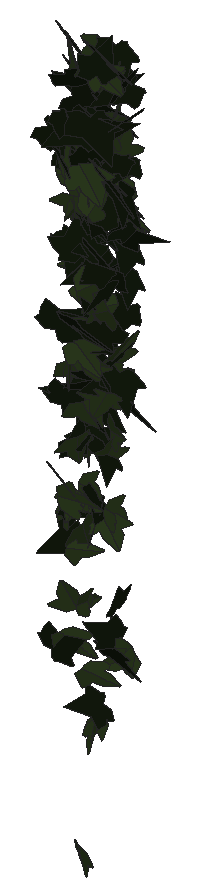
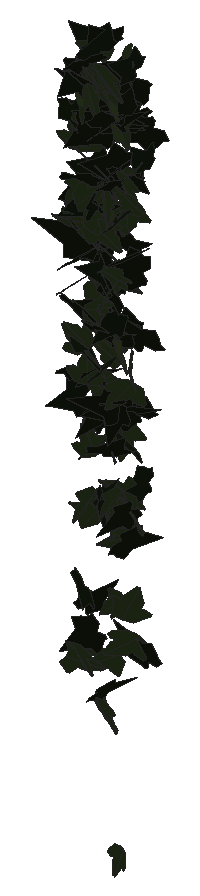
# SketchUp Ruby script. Lengths in inches.
U = 1.inch
M = Sketchup.active_model
def pt(a) = Geom::Point3d.new(a.map { |v| v * U })
def face(e, loops, mat)
  f = e.add_face(loops[0].map { |a| pt(a) })
  loops[1..].each { |l| e.add_face(l.map { |a| pt(a) }).erase! }
  f.material = f.back_material = mat if mat
  f
end
# faces: each face lists its corners as indices into pts; further lists are holes
def faces(e, pts, list, mat = nil) = list.each { |f| face(e, (f[0].is_a?(Array) ? f : [f]).map { |l| l.map { |i| pts[i] } }, mat) }
# xy, xz, yz: faces in a plane at the given z, y or x. An outline is a flat list of corners, or four numbers for a rectangle; further outlines are holes
def ring(l) = l.size == 4 ? [[l[0], l[1]], [l[2], l[1]], [l[2], l[3]], [l[0], l[3]]] : l.each_slice(2).to_a
def flat(e, list, mat, &to3) = list.each { |f| face(e, (f[0].is_a?(Array) ? f : [f]).map { |l| ring(l).map { |u, v| to3.(u, v) } }, mat) }
def xy(e, z, list, mat = nil) = flat(e, list, mat) { |x, y| [x, y, z] }
def xz(e, y, list, mat = nil) = flat(e, list, mat) { |x, z| [x, y, z] }
def yz(e, x, list, mat = nil) = flat(e, list, mat) { |y, z| [x, y, z] }
def lines(e, pts, list) = list.each { |a, b| e.add_line(pt(pts[a]), pt(pts[b])) }
# prism: a flat outline (further loops are holes) pulled along v
def prism(e, loops, v, mat = nil)
  f = face(e, loops, mat); d = Geom::Vector3d.new(v.map { |x| x * U })
  f.pushpull(f.normal.samedirection?(d) ? d.length : -d.length)
end
def box(e, o, s, mat = nil) = prism(e, [[o, [o[0] + s[0], o[1], o[2]], [o[0] + s[0], o[1] + s[1], o[2]], [o[0], o[1] + s[1], o[2]]]], [0, 0, s[2]], mat)
def at(x, y, z, deg = 0) = Geom::Transformation.translation(pt([x, y, z])) * Geom::Transformation.rotation(ORIGIN, Z_AXIS, deg.degrees)
def axes(o, x, y, z) = Geom::Transformation.new([*x, 0, *y, 0, *z, 0, *pt(o).to_a, 1])
def part(name) = M.definitions.add(name)
# library, detail: a bought-in or finely detailed component or shape, given as its bounding box
def library(name, o, s) = part(name).tap { |d| box(d.entities, o, s) }
def detail(e, o, s) = box(e.add_group.entities, o, s)
def put(e, d, t, mat = nil) = e.add_instance(d, t).tap { |i| i.material = mat if mat }
def group(e, t, mat = nil) = e.add_group.tap { |g| g.transformation = t; g.material = mat if mat }.entities
root = M.entities
M.materials.add("1026 AP 7946 SUNNY SIDE UP").color = [254, 231, 186]
M.materials.add("efeu1").color = [18, 25, 13]
M.materials.add("efeu2").color = [43, 57, 29]
c1 = part("ivyleaf_9")
p = [[1.54,2.16,1.25],[1.36,2.04,1.19],[-0.21,0.99,0.68],[-0.71,1.11,0.82],[-0.85,0.86,0.67],[-0.8,0.17,0.21],
  [-0.9,-0.01,0.1],[-0.67,-0.16,-0.02],[-0.08,-0.08,-0.05],[-0.03,-0.6,-0.4],[0.65,-0.88,-0.66],[0.83,-0.6,-0.49],
  [1.29,-0.42,-0.43],[1.8125,-0.07,-0.26],[1.21,0.44,0.15]]
faces(c1.entities,p,[[0,1,2,3,4,5,6,7,8,9,10,11,12,13,14]],"efeu1")
c2 = part("ivyleaf_10")
p = [[0,0.5,-0.03],[-0.0625,2.02,-0.43],[-0.19,2.01,-0.46],[-0.54,1.05,-0.29],[-0.52,0.625,-0.18],[-0.83,0.76,-0.28],
  [-1.16,0.64,-0.33],[-1.15,0.33,-0.24],[-0.77,-0.39,0.02],[-0.3,-0.51,0.16],[0.04,-0.48,0.23],[-0.02,2.01,-0.4375],
  [-0.06,2.01,-0.43],[0.04,-0.49,0.23],[0.67,-0.49,0.14],[1.38,0.36,-0.2],[1.375,0.51,-0.24],[0.81,0.65,-0.19],
  [0.62,0.59,-0.15],[0.6,1.09,-0.28],[0.5,1.23,-0.31]]
faces(c2.entities,p,[[0,1,2,3,4,5,6,7,8,9,10],[11,12,0,13,14,15,16,17,18,19,20]],"efeu2")
put(root,c1,axes([113.27,211.88,254.59],[-0.05004,0.07467,0.25813],[0.2583,-0.19012,0.07888],[0.31902,0.16565,-0.02338]),"1026 AP 7946 SUNNY SIDE UP")
put(root,c2,axes([113.63,212.07,255.59],[-0.29468,-0.15309,-0.11384],[-0.15695,-0.0504,0.24797],[-0.25106,0.21119,-0.0214]),"1026 AP 7946 SUNNY SIDE UP")
put(root,c2,axes([113.6,212.22,265.22],[0.30589,-0.1507,-0.09853],[-0.12709,0.05033,-0.25304],[0.24942,0.21047,-0.0081]),"1026 AP 7946 SUNNY SIDE UP")
put(root,c1,axes([113.29,211.87,258.46],[0.30159,-0.16187,0.03135],[0.01844,-0.03457,-0.25804],[0.25859,0.19124,-0.01816]),"1026 AP 7946 SUNNY SIDE UP")
put(root,c1,axes([113.3,211.93,265.42],[0.08383,-0.17841,0.21618],[0.07856,-0.20497,-0.19289],[0.42714,0.07271,-0.00695]),"1026 AP 7946 SUNNY SIDE UP")
put(root,c1,axes([113.27,212.27,267.75],[0.20315,-0.19062,0.11843],[0.08131,-0.10486,-0.23738],[0.34134,0.13843,-0.01394]),"1026 AP 7946 SUNNY SIDE UP")
put(root,c2,axes([113.24,212.27,264.72],[0.22167,-0.09358,-0.21902],[0.3188,-0.07055,0.1705],[-0.17669,-0.24469,0.03285]),"1026 AP 7946 SUNNY SIDE UP")
put(root,c2,axes([113.625,211.9,265.02],[-0.03111,0.21778,-0.19952],[-0.04804,0.19274,0.22618],[0.45703,0.03508,0.0102]),"1026 AP 7946 SUNNY SIDE UP")
put(root,c2,axes([113.45,212.23,260.65],[-0.26135,-0.14427,-0.15787],[0.19582,0.08871,-0.22588],[0.26564,-0.20734,0.01119]),"1026 AP 7946 SUNNY SIDE UP")
put(root,c1,axes([113.78,212.56,266.45],[-0.05787,0.05868,0.25753],[-0.38787,-0.07709,-0.01925],[0.11031,-0.24029,0.06743]),"1026 AP 7946 SUNNY SIDE UP")
put(root,c2,axes([113.59,212.34,266.46],[0.02658,-0.25701,0.0449],[-0.0011,-0.04518,-0.26558],[0.41028,0.01653,-0.00362]),"1026 AP 7946 SUNNY SIDE UP")
put(root,c1,axes([113.34,211.91,261.54],[-0.15864,0.08613,0.25559],[0.34664,-0.11572,0.13333],[0.2231,0.24104,-0.02541]),"1026 AP 7946 SUNNY SIDE UP")
put(root,c1,axes([113.82,212.31,260.06],[-0.21043,-0.00737,0.21983],[-0.31368,-0.08559,-0.1324],[0.11986,-0.23693,0.03943]),"1026 AP 7946 SUNNY SIDE UP")
put(root,c1,axes([113.5,212.7,265.54],[-0.06622,-0.20645,0.13706],[-0.03746,-0.1321,-0.21782],[0.38537,-0.04832,0.00238]),"1026 AP 7946 SUNNY SIDE UP")
put(root,c2,axes([113.37,212.01,257.55],[0.11479,-0.15018,-0.19142],[0.19594,-0.14081,0.16763],[-0.3193,-0.1404,0.03405]),"1026 AP 7946 SUNNY SIDE UP")
put(root,c2,axes([113.63,212.33,261.53],[0.16132,-0.2266,-0.02126],[-0.03401,0.0114,-0.25572],[0.35598,0.10378,-0.0148]),"1026 AP 7946 SUNNY SIDE UP")
put(root,c1,axes([113.27,212.07,263.2],[0.30243,-0.1217,0.14574],[0.168,-0.09595,-0.2341],[0.24157,0.21908,-0.01965]),"1026 AP 7946 SUNNY SIDE UP")
put(root,c1,axes([113.36,212.45,266.84],[0.09024,-0.15114,0.22857],[0.14243,-0.2036,-0.16757],[0.39855,0.10699,0.00813]),"1026 AP 7946 SUNNY SIDE UP")
put(root,c1,axes([113.45,212.53,264.46],[0.06337,-0.24092,0.07907],[0.02803,-0.07621,-0.25204],[0.39726,0.04381,0.00517]),"1026 AP 7946 SUNNY SIDE UP")
put(root,c1,axes([113.42,211.57,266.09],[0.06896,0.01598,-0.27906],[0.08466,0.26852,0.02686],[0.41833,-0.05697,0.04056]),"1026 AP 7946 SUNNY SIDE UP")
put(root,c1,axes([113.64,212.37,260.22],[0.31328,-0.00666,-0.15655],[-0.23905,-0.01452,-0.20482],[-0.00554,0.25013,-0.01459]),"1026 AP 7946 SUNNY SIDE UP")
put(root,c1,axes([113.7,212.05,257.125],[0.00686,-0.10836,-0.27003],[0.09102,-0.25566,0.10864],[-0.43568,-0.05512,0.01845]),"1026 AP 7946 SUNNY SIDE UP")
put(root,c2,axes([113.84,211.79,267.53],[-0.08352,0.08772,-0.29124],[-0.17598,0.2605,0.10627],[0.43169,0.12316,-0.01303]),"1026 AP 7946 SUNNY SIDE UP")
put(root,c2,axes([113.7,212,264.4],[-0.37137,-0.10293,-0.00003],[0.01359,-0.02122,-0.26449],[0.16127,-0.23523,0.02222]),"1026 AP 7946 SUNNY SIDE UP")
put(root,c2,axes([113.9375,212.17,262.93],[-0.10002,0.0419,0.23465],[-0.34842,-0.07891,-0.0493],[0.10464,-0.22269,0.06011]),"1026 AP 7946 SUNNY SIDE UP")
put(root,c1,axes([113.6,212,257.8],[0.07037,-0.02062,-0.25548],[-0.11456,0.23972,-0.03269],[0.37396,0.07732,0.03806]),"1026 AP 7946 SUNNY SIDE UP")
put(root,c1,axes([113.62,212.17,263.4],[-0.13101,-0.22908,0.09166],[-0.0102,-0.09322,-0.25043],[0.38703,-0.08,0.02442]),"1026 AP 7946 SUNNY SIDE UP")
put(root,c2,axes([113.61,212.18,264.29],[-0.01572,-0.05606,0.26335],[0.14029,-0.24155,-0.05233],[0.38737,0.08521,0.02964]),"1026 AP 7946 SUNNY SIDE UP")
put(root,c1,axes([113.56,212.19,265.27],[-0.21319,-0.11264,-0.17533],[0.22079,0.09573,-0.18064],[0.23172,-0.19485,0.01081]),"1026 AP 7946 SUNNY SIDE UP")
put(root,c2,axes([113.65,212.4375,266.98],[0.13269,-0.19606,0.17999],[0.08969,-0.16664,-0.2206],[0.40426,0.10132,-0.01014]),"1026 AP 7946 SUNNY SIDE UP")
put(root,c2,axes([113.52,212.03,260.88],[0.13338,-0.1309,0.24849],[0.25586,-0.18027,-0.1603],[0.34875,0.18231,0.02257]),"1026 AP 7946 SUNNY SIDE UP")
put(root,c1,axes([113.58,212.3,265.2],[-0.03379,-0.28354,-0.06617],[0.01587,0.06202,-0.29252],[0.4563,-0.02315,0.00527]),"1026 AP 7946 SUNNY SIDE UP")
put(root,c1,axes([113.48,211.91,259.96],[-0.08664,0.04162,0.2526],[0.34837,-0.10536,0.06917],[0.17688,0.22791,-0.01249]),"1026 AP 7946 SUNNY SIDE UP")
put(root,c2,axes([113.75,212.52,264.82],[0.06468,-0.23733,-0.09699],[0.00366,0.09435,-0.24696],[0.40068,0.03745,0.01791]),"1026 AP 7946 SUNNY SIDE UP")
put(root,c1,axes([113.5,212.12,260.1],[0.22925,0.09403,0.21067],[0.27717,0.10278,-0.17802],[-0.21884,0.22867,-0.00478]),"1026 AP 7946 SUNNY SIDE UP")
put(root,c2,axes([113.92,212.59,264.17],[-0.25604,-0.09566,0.17523],[-0.19915,-0.11765,-0.19315],[0.23442,-0.20443,0.02731]),"1026 AP 7946 SUNNY SIDE UP")
put(root,c1,axes([113.84,211.79,259.18],[-0.27709,0.15901,-0.09797],[-0.09756,0.07434,0.24461],[0.27529,0.1864,-0.01192]),"1026 AP 7946 SUNNY SIDE UP")
put(root,c1,axes([113.64,211.69,266.43],[0.10789,-0.08843,-0.24258],[-0.09764,0.23004,-0.10652],[0.3825,0.08367,0.04123]),"1026 AP 7946 SUNNY SIDE UP")
put(root,c2,axes([113.57,211.9375,254.93],[-0.27349,-0.07845,-0.18939],[0.2844,0.04058,-0.19436],[0.13226,-0.24948,0.0263]),"1026 AP 7946 SUNNY SIDE UP")
put(root,c2,axes([113.75,212.11,250.25],[-0.27635,0.16463,-0.00203],[-0.01617,-0.01522,-0.24747],[-0.2584,-0.17511,0.01766]),"1026 AP 7946 SUNNY SIDE UP")
put(root,c2,axes([113.92,212.48,267.57],[0.31323,-0.13901,-0.15376],[-0.2093,0.06801,-0.2492],[0.24179,0.23895,-0.01653]),"1026 AP 7946 SUNNY SIDE UP")
put(root,c1,axes([113.96,211.93,266.09],[-0.3323,-0.10845,0.11137],[-0.11543,-0.0911,-0.24116],[0.21208,-0.21951,0.04324]),"1026 AP 7946 SUNNY SIDE UP")
put(root,c2,axes([113.76,211.89,258.05],[0.36123,-0.07041,0.01554],[0.01298,-0.02567,-0.24664],[0.11262,0.22882,-0.0214]),"1026 AP 7946 SUNNY SIDE UP")
put(root,c1,axes([113.98,212.33,259.1],[-0.3356,-0.13268,0.05508],[0.05564,0.04547,0.25838],[-0.21839,0.21546,-0.01881]),"1026 AP 7946 SUNNY SIDE UP")
put(root,c2,axes([113.8,212.18,258.15],[-0.04496,0.19723,0.19435],[-0.0427,0.18555,-0.20422],[-0.4258,-0.03944,-0.00004]),"1026 AP 7946 SUNNY SIDE UP")
put(root,c1,axes([113.75,212.64,266.39],[-0.08165,-0.21696,0.12473],[-0.02237,-0.12215,-0.23016],[0.39099,-0.0523,0.01288]),"1026 AP 7946 SUNNY SIDE UP")
put(root,c1,axes([113.52,212.38,260.25],[0.20957,0.01948,0.22086],[0.3337,0.02957,-0.13859],[-0.05566,0.2506,0.00068]),"1026 AP 7946 SUNNY SIDE UP")
put(root,c2,axes([113.76,212.4,264.36],[0.2108,-0.16853,0.13734],[0.12707,-0.10727,-0.22246],[0.31409,0.15651,-0.00218]),"1026 AP 7946 SUNNY SIDE UP")
put(root,c1,axes([113.68,211.8,267.2],[0.38482,0.16159,0.06805],[0.10007,0.02164,-0.30151],[-0.25501,0.25232,-0.01563]),"1026 AP 7946 SUNNY SIDE UP")
put(root,c1,axes([113.72,212.17,262.15],[0.39523,-0.11676,-0.0876],[-0.13853,0.00963,-0.28409],[0.1792,0.26496,-0.02642]),"1026 AP 7946 SUNNY SIDE UP")
put(root,c2,axes([113.94,212.59,264.22],[-0.13393,-0.17633,-0.16859],[-0.13735,-0.13795,0.20039],[-0.35131,0.12116,-0.01407]),"1026 AP 7946 SUNNY SIDE UP")
put(root,c2,axes([113.875,212.01,255.69],[0.04459,0.01048,0.24675],[-0.06063,0.23819,-0.00464],[-0.37198,-0.03757,0.03034]),"1026 AP 7946 SUNNY SIDE UP")
put(root,c2,axes([114.05,212.01,261.76],[-0.32387,-0.07909,0.11847],[-0.15,-0.07095,-0.22582],[0.161,-0.22521,0.02793]),"1026 AP 7946 SUNNY SIDE UP")
put(root,c2,axes([113.92,211.77,259.36],[-0.16478,-0.25487,-0.06279],[0.04743,0.05191,-0.28347],[0.4088,-0.10876,0.00758]),"1026 AP 7946 SUNNY SIDE UP")
put(root,c2,axes([113.95,212.02,262.49],[-0.00201,0.26876,0.03596],[-0.01811,-0.0334,0.27642],[0.42545,-0.00015,0.01193]),"1026 AP 7946 SUNNY SIDE UP")
put(root,c1,axes([113.76,212.28,264.04],[0.22277,-0.18775,-0.11347],[-0.05521,0.10872,-0.23913],[0.33693,0.14195,0.03584]),"1026 AP 7946 SUNNY SIDE UP")
put(root,c1,axes([114.01,211.8,263.44],[-0.38661,-0.03742,0.11688],[0.17411,0.02733,0.25619],[-0.07135,0.26949,-0.00813]),"1026 AP 7946 SUNNY SIDE UP")
put(root,c1,axes([113.83,211.82,266.79],[0.03282,0.06007,-0.25975],[-0.03559,0.25275,0.0615],[0.40652,0.01728,0.02636]),"1026 AP 7946 SUNNY SIDE UP")
put(root,c1,axes([113.62,211.96,261.66],[0.21546,-0.11644,0.19895],[0.24236,-0.11765,-0.1858],[0.26006,0.20612,0.00832]),"1026 AP 7946 SUNNY SIDE UP")
put(root,c2,axes([113.64,211.8,257.99],[-0.06814,0.02611,0.27857],[0.4207,0.05069,0.03945],[-0.07267,0.26898,-0.03283]),"1026 AP 7946 SUNNY SIDE UP")
put(root,c2,axes([114,211.98,264.51],[0.05328,-0.02949,-0.27694],[0.01878,0.27066,-0.02748],[0.42456,-0.00827,0.03597]),"1026 AP 7946 SUNNY SIDE UP")
put(root,c2,axes([114.07,211.89,264.48],[0.03061,-0.13039,-0.24809],[-0.06834,0.23615,-0.13437],[0.42412,0.04746,-0.00375]),"1026 AP 7946 SUNNY SIDE UP")
put(root,c1,axes([113.83,212,265.25],[0.04058,0.05468,0.2931],[0.34226,0.18438,-0.05583],[-0.29992,0.21781,-0.02405]),"1026 AP 7946 SUNNY SIDE UP")
put(root,c1,axes([113.77,212.29,262.68],[-0.06293,-0.04935,-0.24773],[0.38549,-0.01306,-0.0394],[-0.00793,-0.24315,0.05091]),"1026 AP 7946 SUNNY SIDE UP")
put(root,c1,axes([113.88,212.4,263.98],[-0.02506,-0.16502,0.23019],[-0.00627,-0.22459,-0.17176],[0.43791,-0.01266,0.01072]),"1026 AP 7946 SUNNY SIDE UP")
put(root,c2,axes([113.85,211.76,257.02],[-0.01927,-0.06563,-0.23881],[0.25781,0.1673,-0.05684],[0.27681,-0.16039,0.03632]),"1026 AP 7946 SUNNY SIDE UP")
put(root,c2,axes([113.875,212.17,259.17],[0.07499,-0.09191,0.23542],[0.24243,-0.17106,-0.10479],[0.30301,0.15961,0.02558]),"1026 AP 7946 SUNNY SIDE UP")
put(root,c2,axes([114.35,212.26,267.2],[-0.1237,0.07956,0.25999],[-0.38789,0.07195,-0.10235],[-0.14868,-0.25392,0.05071]),"1026 AP 7946 SUNNY SIDE UP")
put(root,c1,axes([114.14,212.28,263.41],[-0.20788,-0.07327,0.21479],[-0.12097,-0.21296,-0.12834],[0.32641,-0.12558,0.08923]),"1026 AP 7946 SUNNY SIDE UP")
put(root,c2,axes([114.1,211.72,257.59],[-0.06356,-0.26306,-0.15209],[0.04628,0.14329,-0.27326],[0.4709,-0.04958,0.00633]),"1026 AP 7946 SUNNY SIDE UP")
put(root,c1,axes([113.91,212.4,260.98],[0.08493,-0.24193,0.05168],[0.01667,-0.05044,-0.25566],[0.38858,0.05504,-0.00033]),"1026 AP 7946 SUNNY SIDE UP")
put(root,c1,axes([114.05,211.92,262.65],[0.14438,-0.13704,-0.19892],[-0.18734,0.15126,-0.16876],[0.32058,0.15011,-0.00903]),"1026 AP 7946 SUNNY SIDE UP")
put(root,c1,axes([113.99,212.25,259.98],[0.03826,-0.11868,-0.22909],[-0.04096,0.22035,-0.12318],[0.39328,0.0345,0.00946]),"1026 AP 7946 SUNNY SIDE UP")
put(root,c2,axes([114.05,211.86,260.125],[-0.29432,-0.17813,-0.12219],[0.1532,0.06786,-0.26526],[0.29861,-0.21038,0.01566]),"1026 AP 7946 SUNNY SIDE UP")
put(root,c2,axes([114.24,212.65,264.71],[-0.06127,-0.0692,-0.25102],[-0.20143,-0.20684,0.08054],[-0.34291,0.13386,-0.00246]),"1026 AP 7946 SUNNY SIDE UP")
put(root,c1,axes([114.02,211.93,262.8],[-0.02713,0.23321,-0.13084],[-0.01229,0.1281,0.24165],[0.41838,0.01888,-0.00138]),"1026 AP 7946 SUNNY SIDE UP")
put(root,c2,axes([114.23,212.38,262.16],[-0.08002,0.0174,0.25628],[-0.06164,-0.2512,0.00837],[0.38708,-0.0364,0.05432]),"1026 AP 7946 SUNNY SIDE UP")
put(root,c2,axes([114.12,212.12,262.15],[-0.06523,0.12831,0.21702],[0.09429,-0.2012,0.13772],[0.3752,0.07287,0.00312]),"1026 AP 7946 SUNNY SIDE UP")
put(root,c1,axes([114.29,212.19,261.67],[-0.37726,-0.01428,-0.0338],[0.0533,-0.02129,-0.24659],[0.01763,-0.24121,0.02233]),"1026 AP 7946 SUNNY SIDE UP")
put(root,c1,axes([114.03,212.26,259.68],[-0.04649,-0.09187,0.24917],[0.05692,-0.24304,-0.09177],[0.4036,0.02369,0.04164]),"1026 AP 7946 SUNNY SIDE UP")
put(root,c1,axes([113.97,212.38,266.3],[0.39907,0.04217,0.03452],[0.05621,-0.01269,-0.26445],[-0.06303,0.25565,-0.01728]),"1026 AP 7946 SUNNY SIDE UP")
put(root,c2,axes([114.28,212.03,253.32],[0.26277,-0.15517,-0.12085],[-0.14824,0.06934,-0.23421],[0.26659,0.1915,-0.01112]),"1026 AP 7946 SUNNY SIDE UP")
put(root,c2,axes([114.21,212.44,267.01],[-0.00487,-0.26235,0.0016],[0.00534,-0.00308,-0.27029],[0.41252,-0.00306,0.00351]),"1026 AP 7946 SUNNY SIDE UP")
put(root,c1,axes([114.26,212.09,253.62],[0.04029,-0.18535,-0.18064],[0.03616,-0.17277,0.19175],[-0.39842,-0.03443,-0.00087]),"1026 AP 7946 SUNNY SIDE UP")
put(root,c2,axes([113.99,211.88,265.15],[0.33798,0.16461,0.12151],[0.16079,0.05865,-0.27818],[-0.27385,0.2376,-0.01337]),"1026 AP 7946 SUNNY SIDE UP")
put(root,c2,axes([114.09,211.73,262.77],[0.05713,0.00667,-0.31089],[0.20076,0.27513,0.02371],[0.43015,-0.12929,0.03022]),"1026 AP 7946 SUNNY SIDE UP")
put(root,c1,axes([114.16,212.2,257.87],[-0.17698,0.05259,-0.2647],[0.32836,-0.15172,-0.12697],[-0.25025,-0.23627,0.0206]),"1026 AP 7946 SUNNY SIDE UP")
put(root,c1,axes([114.49,212.21,264.25],[-0.34877,-0.11412,-0.0566],[-0.0922,-0.00423,0.2559],[-0.17603,0.22831,-0.02188]),"1026 AP 7946 SUNNY SIDE UP")
put(root,c2,axes([114.18,211.85,264.43],[0.13025,0.13704,-0.23674],[0.10823,0.22239,0.16293],[0.40764,-0.10283,0.03239]),"1026 AP 7946 SUNNY SIDE UP")
put(root,c2,axes([114.01,211.73,261.41],[0.28779,0.09439,0.16013],[0.22521,0.05983,-0.21155],[-0.17502,0.23219,-0.00891]),"1026 AP 7946 SUNNY SIDE UP")
put(root,c1,axes([114.14,212.15,257.97],[-0.03507,-0.17301,0.19113],[0.00377,-0.18736,-0.17985],[0.40001,-0.0134,0.01845]),"1026 AP 7946 SUNNY SIDE UP")
put(root,c2,axes([114.15,211.97,253.17],[0.22699,-0.14547,0.15194],[0.14231,-0.11853,-0.21121],[0.29404,0.16967,-0.01507]),"1026 AP 7946 SUNNY SIDE UP")
put(root,c2,axes([114.01,211.95,260.98],[-0.15963,0.01137,0.22098],[0.33765,0.00419,0.10452],[0.00169,0.23722,-0.01104]),"1026 AP 7946 SUNNY SIDE UP")
put(root,c1,axes([114.61,211.9,261.71],[-0.13306,0.06686,0.26944],[-0.36825,0.11734,-0.10844],[-0.20994,-0.24819,0.01943]),"1026 AP 7946 SUNNY SIDE UP")
put(root,c2,axes([114.53,211.89,262.33],[-0.26051,0.06563,0.22477],[-0.33728,0.04465,-0.18169],[-0.1191,-0.26999,0.02287]),"1026 AP 7946 SUNNY SIDE UP")
put(root,c1,axes([114.52,211.87,263.31],[-0.41901,0.11303,0.00247],[-0.01856,-0.02334,-0.29712],[-0.17678,-0.26546,0.02533]),"1026 AP 7946 SUNNY SIDE UP")
put(root,c1,axes([113.93,211.875,266.02],[0.0126,0.03614,0.32054],[0.48591,-0.05053,-0.00245],[0.07852,0.30691,-0.03628]),"1026 AP 7946 SUNNY SIDE UP")
put(root,c1,axes([114.32,212.7,265.23],[-0.30535,-0.14435,-0.00977],[0.03462,-0.01518,-0.24799],[0.22474,-0.19379,0.02493]),"1026 AP 7946 SUNNY SIDE UP")
put(root,c2,axes([114.1,211.92,254.36],[-0.16125,-0.09549,-0.21592],[0.29487,0.09757,-0.14011],[0.20892,-0.21141,0.03111]),"1026 AP 7946 SUNNY SIDE UP")
put(root,c2,axes([114.3125,212.38,260.66],[-0.27978,-0.1741,-0.01203],[-0.03108,0.00496,0.25586],[-0.2725,0.17818,-0.01684]),"1026 AP 7946 SUNNY SIDE UP")
put(root,c2,axes([114.45,212.31,266.29],[-0.1984,-0.19483,0.12527],[-0.09239,-0.10804,-0.2396],[0.35006,-0.13894,0.00776]),"1026 AP 7946 SUNNY SIDE UP")
put(root,c1,axes([114.43,212.31,260.54],[-0.15911,-0.10087,0.21672],[-0.20658,-0.16561,-0.14748],[0.30414,-0.16526,0.01321]),"1026 AP 7946 SUNNY SIDE UP")
put(root,c1,axes([114.17,211.91,266.37],[-0.15373,-0.19472,-0.1925],[0.15811,0.15689,-0.22302],[0.3925,-0.13946,0.01444]),"1026 AP 7946 SUNNY SIDE UP")
put(root,c1,axes([114.11,212.56,264.67],[0.34313,-0.10357,0.01386],[0.00783,-0.02217,-0.24829],[0.16415,0.21755,-0.01713]),"1026 AP 7946 SUNNY SIDE UP")
put(root,c2,axes([114.44,211.97,260.41],[-0.31764,-0.14201,0.08324],[-0.08224,-0.06685,-0.25364],[0.24406,-0.20736,0.02286]),"1026 AP 7946 SUNNY SIDE UP")
put(root,c2,axes([114.06,212.27,267.05],[0.27441,-0.09104,-0.19724],[0.28464,-0.0638,0.20141],[-0.1721,-0.25069,0.01861]),"1026 AP 7946 SUNNY SIDE UP")
put(root,c2,axes([114.3125,212.4,267.37],[0.27772,-0.20323,0.05979],[0.04258,-0.05476,-0.27726],[0.33009,0.17804,-0.01454]),"1026 AP 7946 SUNNY SIDE UP")
put(root,c2,axes([114.52,212.58,254.49],[0.14662,0.05944,-0.22499],[-0.2856,-0.12189,-0.11461],[-0.21321,0.20416,-0.0012]),"1026 AP 7946 SUNNY SIDE UP")
put(root,c1,axes([114.26,212.24,259.0625],[-0.01379,-0.23106,0.10358],[0.00617,-0.10203,-0.23869],[0.39701,-0.00644,0.00731]),"1026 AP 7946 SUNNY SIDE UP")
put(root,c2,axes([114.35,212.22,259.01],[-0.11332,-0.24022,0.03294],[0.00451,0.03393,0.25847],[-0.38132,0.07179,-0.00673]),"1026 AP 7946 SUNNY SIDE UP")
put(root,c2,axes([114.49,212.53,254.69],[0.29057,-0.11757,-0.11116],[-0.15165,0.04797,-0.22511],[0.19903,0.2082,-0.00924]),"1026 AP 7946 SUNNY SIDE UP")
put(root,c1,axes([114.27,212.52,267.7],[-0.04697,-0.25864,-0.04761],[0.01742,0.04376,-0.26789],[0.41236,-0.03131,0.0059]),"1026 AP 7946 SUNNY SIDE UP")
put(root,c1,axes([114.56,211.93,262.99],[0.20771,-0.10845,0.22953],[-0.23764,0.16571,0.17589],[-0.30988,-0.19977,0.01898]),"1026 AP 7946 SUNNY SIDE UP")
put(root,c2,axes([114.49,212.27,265.86],[-0.18505,0.24272,-0.03038],[-0.01494,0.02969,0.27803],[0.38444,0.11799,-0.00382]),"1026 AP 7946 SUNNY SIDE UP")
put(root,c2,axes([114.32,212.4375,264.93],[0.09769,0.19188,0.15661],[0.07892,0.14238,-0.20692],[-0.37567,0.07981,-0.00275]),"1026 AP 7946 SUNNY SIDE UP")
put(root,c2,axes([114.43,212.47,266.64],[-0.11119,0.08894,-0.2303],[-0.00576,-0.23387,-0.09582],[-0.37901,-0.02254,0.06902]),"1026 AP 7946 SUNNY SIDE UP")
put(root,c2,axes([114.46,212.125,257.86],[-0.01629,0.1778,0.22016],[-0.05999,0.2099,-0.18146],[-0.43176,-0.03587,0.0169]),"1026 AP 7946 SUNNY SIDE UP")
put(root,c1,axes([114.39,212.74,263.36],[-0.07253,-0.22788,0.09057],[-0.01324,-0.08925,-0.23987],[0.38458,-0.04605,0.00883]),"1026 AP 7946 SUNNY SIDE UP")
put(root,c2,axes([114.27,212.15,257.61],[0.33664,0.12292,0.11659],[0.17341,0.03274,-0.25292],[-0.19639,0.23962,-0.02346]),"1026 AP 7946 SUNNY SIDE UP")
put(root,c1,axes([114.61,212.13,255.85],[-0.00074,0.1625,0.2063],[-0.00101,0.19933,-0.16625],[-0.40439,-0.0008,0.00004]),"1026 AP 7946 SUNNY SIDE UP")
put(root,c1,axes([114.68,212.22,261.35],[-0.20122,0.21906,-0.03721],[0.01166,-0.03888,-0.26124],[-0.34923,-0.12751,0.01271]),"1026 AP 7946 SUNNY SIDE UP")
put(root,c1,axes([114.7,212.29,265.54],[-0.35211,0.09549,-0.02852],[0.02781,-0.03021,-0.25006],[-0.15408,-0.22367,0.02003]),"1026 AP 7946 SUNNY SIDE UP")
put(root,c2,axes([114.5,212.27,265.71],[-0.37251,-0.15487,0.05454],[0.05064,0.04878,0.29092],[-0.25278,0.238,-0.0221]),"1026 AP 7946 SUNNY SIDE UP")
put(root,c1,axes([114.41,212.68,262.81],[-0.03203,-0.2462,0.07392],[0.00992,-0.07384,-0.25464],[0.40373,-0.01772,0.01212]),"1026 AP 7946 SUNNY SIDE UP")
put(root,c1,axes([114.28,212.46,264.69],[-0.07875,-0.06025,-0.27879],[0.42187,0.05742,-0.06407],[0.10776,-0.26882,0.04708]),"1026 AP 7946 SUNNY SIDE UP")
put(root,c1,axes([114.53,211.62,267.6],[-0.20474,-0.06155,0.22888],[0.2742,0.14121,0.14619],[-0.23792,0.21571,-0.02848]),"1026 AP 7946 SUNNY SIDE UP")
put(root,c1,axes([114.59,212.46,262.21],[-0.3588,-0.01983,-0.12765],[0.19684,-0.0217,-0.23425],[0.011,-0.2587,0.0279]),"1026 AP 7946 SUNNY SIDE UP")
put(root,c1,axes([114.28,212.14,265.1],[0.21133,-0.23276,0.15028],[0.11448,-0.12793,-0.27764],[0.41763,0.15285,0.00006]),"1026 AP 7946 SUNNY SIDE UP")
put(root,c1,axes([114.69,211.92,255.3],[0.01281,0.02614,0.25067],[-0.30166,-0.15022,0.02238],[0.23851,-0.1914,0.01484]),"1026 AP 7946 SUNNY SIDE UP")
put(root,c1,axes([114.38,212.08,254.9],[0.39319,-0.04645,0.00456],[0.00057,-0.02362,-0.26107],[0.07341,0.24899,-0.02239]),"1026 AP 7946 SUNNY SIDE UP")
put(root,c1,axes([114.79,212.34,267.13],[-0.41725,0.00265,0.01553],[-0.02397,-0.0254,-0.27227],[-0.00188,-0.26457,0.02473]),"1026 AP 7946 SUNNY SIDE UP")
put(root,c1,axes([114.45,212.39,264.66],[0.03063,-0.22743,0.12469],[0.00869,-0.12228,-0.23583],[0.40597,0.01978,-0.00436]),"1026 AP 7946 SUNNY SIDE UP")
put(root,c1,axes([114.8,212.33,264.08],[-0.2706,0.16707,-0.03528],[0.022,-0.036,-0.24676],[-0.26757,-0.17192,0.01539]),"1026 AP 7946 SUNNY SIDE UP")
put(root,c1,axes([114.52,212.34,260.76],[-0.13527,-0.22279,-0.09393],[0.07124,0.07875,-0.24521],[0.371,-0.09635,0.01283]),"1026 AP 7946 SUNNY SIDE UP")
put(root,c2,axes([114.34,212.54,264.1],[-0.09861,-0.07157,-0.22795],[0.35322,-0.07652,-0.04061],[-0.09227,-0.21647,0.08816]),"1026 AP 7946 SUNNY SIDE UP")
put(root,c1,axes([114.26,212.46,263.71],[0.26277,0.10731,-0.2013],[0.2349,0.12838,0.20437],[0.26132,-0.22331,0.01872]),"1026 AP 7946 SUNNY SIDE UP")
put(root,c1,axes([114.76,212.28,266.42],[-0.07165,0.24208,-0.03711],[0.00471,-0.03748,-0.25396],[-0.38514,-0.04549,0.0038]),"1026 AP 7946 SUNNY SIDE UP")
put(root,c1,axes([114.74,211.82,263.07],[-0.32173,0.14597,-0.16002],[0.17769,-0.10962,-0.25875],[-0.2853,-0.23288,0.0193]),"1026 AP 7946 SUNNY SIDE UP")
put(root,c1,axes([114.33,212.02,267.71],[0.08628,-0.17978,0.23512],[0.23077,-0.18445,-0.18629],[0.39572,0.14677,0.05738]),"1026 AP 7946 SUNNY SIDE UP")
put(root,c1,axes([114.71,212.14,267.13],[-0.10417,0.11533,-0.27356],[-0.22372,0.22504,0.13824],[0.39754,0.15686,0.00611]),"1026 AP 7946 SUNNY SIDE UP")
put(root,c2,axes([114.58,212.22,261.25],[-0.0178,-0.24267,0.13904],[0.02106,0.13583,0.25098],[-0.43717,0.01642,0.00643]),"1026 AP 7946 SUNNY SIDE UP")
put(root,c1,axes([114.4,212.4375,260.22],[0.34424,-0.10603,0.05303],[0.05872,-0.04192,-0.24991],[0.17622,0.2211,-0.02031]),"1026 AP 7946 SUNNY SIDE UP")
put(root,c2,axes([114.4375,212.2,259.53],[-0.12154,0.06921,0.24037],[0.32499,-0.1098,0.10363],[0.20092,0.21948,-0.02222]),"1026 AP 7946 SUNNY SIDE UP")
put(root,c2,axes([114.51,211.74,267.55],[0.17534,0.17459,0.16882],[0.09908,0.15188,-0.21127],[-0.36214,0.12609,0.02393]),"1026 AP 7946 SUNNY SIDE UP")
